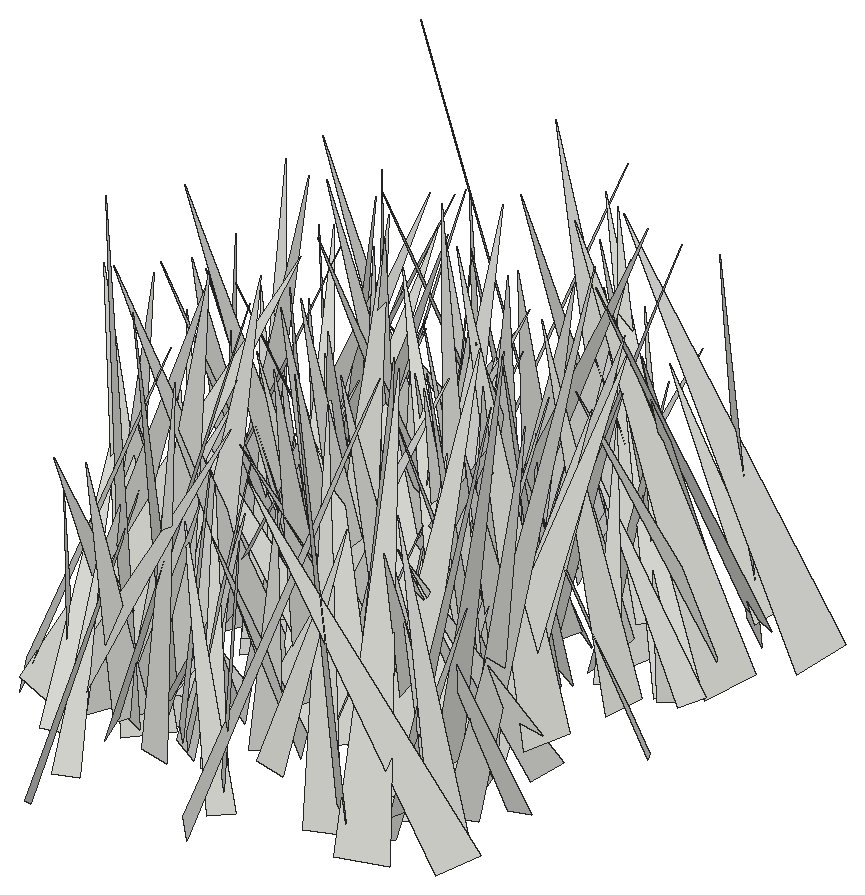
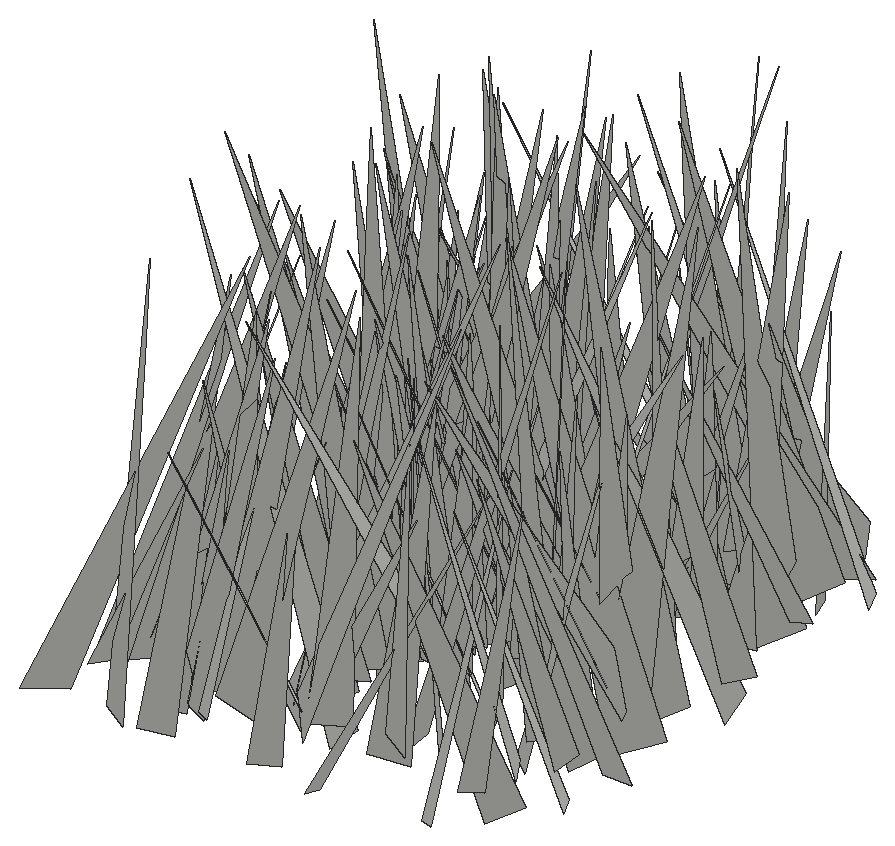
# SketchUp Ruby script. Lengths in inches.
U = 1.inch
M = Sketchup.active_model
def pt(a) = Geom::Point3d.new(a.map { |v| v * U })
def face(e, loops, mat)
  f = e.add_face(loops[0].map { |a| pt(a) })
  loops[1..].each { |l| e.add_face(l.map { |a| pt(a) }).erase! }
  f.material = f.back_material = mat if mat
  f
end
# faces: each face lists its corners as indices into pts; further lists are holes
def faces(e, pts, list, mat = nil) = list.each { |f| face(e, (f[0].is_a?(Array) ? f : [f]).map { |l| l.map { |i| pts[i] } }, mat) }
# xy, xz, yz: faces in a plane at the given z, y or x. An outline is a flat list of corners, or four numbers for a rectangle; further outlines are holes
def ring(l) = l.size == 4 ? [[l[0], l[1]], [l[2], l[1]], [l[2], l[3]], [l[0], l[3]]] : l.each_slice(2).to_a
def flat(e, list, mat, &to3) = list.each { |f| face(e, (f[0].is_a?(Array) ? f : [f]).map { |l| ring(l).map { |u, v| to3.(u, v) } }, mat) }
def xy(e, z, list, mat = nil) = flat(e, list, mat) { |x, y| [x, y, z] }
def xz(e, y, list, mat = nil) = flat(e, list, mat) { |x, z| [x, y, z] }
def yz(e, x, list, mat = nil) = flat(e, list, mat) { |y, z| [x, y, z] }
def lines(e, pts, list) = list.each { |a, b| e.add_line(pt(pts[a]), pt(pts[b])) }
# prism: a flat outline (further loops are holes) pulled along v
def prism(e, loops, v, mat = nil)
  f = face(e, loops, mat); d = Geom::Vector3d.new(v.map { |x| x * U })
  f.pushpull(f.normal.samedirection?(d) ? d.length : -d.length)
end
def box(e, o, s, mat = nil) = prism(e, [[o, [o[0] + s[0], o[1], o[2]], [o[0] + s[0], o[1] + s[1], o[2]], [o[0], o[1] + s[1], o[2]]]], [0, 0, s[2]], mat)
def at(x, y, z, deg = 0) = Geom::Transformation.translation(pt([x, y, z])) * Geom::Transformation.rotation(ORIGIN, Z_AXIS, deg.degrees)
def axes(o, x, y, z) = Geom::Transformation.new([*x, 0, *y, 0, *z, 0, *pt(o).to_a, 1])
def part(name) = M.definitions.add(name)
# library, detail: a bought-in or finely detailed component or shape, given as its bounding box
def library(name, o, s) = part(name).tap { |d| box(d.entities, o, s) }
def detail(e, o, s) = box(e.add_group.entities, o, s)
def put(e, d, t, mat = nil) = e.add_instance(d, t).tap { |i| i.material = mat if mat }
def group(e, t, mat = nil) = e.add_group.tap { |g| g.transformation = t; g.material = mat if mat }.entities
root = M.entities
c1 = part("fur_instance\#9")
p = [[0.8125,0,1.79],[0.67,-0.02,1.48],[0,-0.11,0],[0,0.11,0]]
faces(c1.entities,p,[[0,1,2,3]])
put(root,c1,axes([142.4,106.45,-27.1],[-2.65775,-2.55388,1.91088],[-2.80676,3.05414,0.17806],[1.51521,1.17784,3.68161]))
put(root,c1,axes([137.93,107.84,-27.1],[3.7662,-3.06911,1.25827],[-2.92554,-3.97067,-0.92842],[-1.56328,0.03677,4.76883]))
put(root,c1,axes([137.35,105.55,-28.22],[-2.23531,2.8422,0.49749],[2.78374,2.28983,-0.57415],[0.75919,-0.0278,3.57002]))
put(root,c1,axes([137.45,103.67,-28.22],[4.27823,3.00126,0.70858],[2.21616,-3.83495,2.86263],[-2.14435,2.02448,4.3722]))
put(root,c1,axes([136.09,107.46,-28.22],[-3.74193,-1.93414,1.83822],[-1.95383,4.14237,0.38123],[1.81727,0.47108,4.19495]))
put(root,c1,axes([136.15,106.62,-27.1],[3.52755,5.08967,0.59914],[4.90233,-3.13928,-2.19532],[1.49362,-1.71683,5.79042]))
put(root,c1,axes([139.86,106.47,-27.1],[1.56528,5.39191,1.82425],[5.61252,-1.77733,0.43748],[-0.9488,-1.61836,5.59744]))
put(root,c1,axes([146.14,107.22,-27.1],[3.85266,4.81198,3.39076],[5.17881,-4.69725,0.78179],[-2.79863,-2.06788,6.11449]))
put(root,c1,axes([149.42,108.47,-28.22],[-4.43221,4.72995,1.58971],[4.78005,3.41433,3.16821],[-1.43205,-3.24253,5.65503]))
put(root,c1,axes([142.23,106.57,-28.22],[-1.14245,4.14217,0.46464],[4.01441,0.96381,1.27839],[-1.12161,-0.76952,4.10226]))
put(root,c1,axes([141.9375,105.26,-28.22],[5.64336,5.1887,0.30355],[5.15395,-5.64438,0.66329],[-0.67191,0.28398,7.63742]))
put(root,c1,axes([138.24,109.37,-27.1],[-6.05203,-3.65216,2.90127],[-3.20675,6.70926,1.75646],[3.38709,-0.1736,6.84691]))
put(root,c1,axes([142.83,109.61,-27.1],[-3.8372,-2.33717,0.79383],[-2.01321,3.81242,1.493],[1.42812,-0.90538,4.23762]))
put(root,c1,axes([136.82,105.87,-27.1],[-2.17484,4.53028,0.06229],[4.50087,2.16823,-0.54601],[0.51907,0.1805,4.99552]))
put(root,c1,axes([133.94,107.85,-27.1],[5.98281,3.47845,0.55141],[3.51313,-5.81778,-1.41742],[0.2481,-1.50052,6.77381]))
put(root,c1,axes([137.92,106.97,-27.1],[6.78168,2.91502,1.19431],[2.8839,-6.88568,0.43057],[-1.26762,-0.07012,7.36906]))
put(root,c1,axes([136.63,110.59,-28.22],[3.41213,-4.67618,0.33772],[-4.46229,-3.36731,-1.54031],[-1.43828,-0.64649,5.58003]))
put(root,c1,axes([139.65,107.97,-27.1],[3.10895,3.01642,1.49943],[3.22004,-3.26039,-0.11754],[-0.98914,-1.13301,4.33019]))
put(root,c1,axes([140.05,107.74,-27.1],[3.54809,3.00738,1.07129],[3.07779,-3.64774,0.04651],[-0.84804,-0.65624,4.65093]))
put(root,c1,axes([147.12,106.93,-28.22],[-2.63415,6.93544,1.64719],[7.09873,2.71215,-0.06728],[0.64926,-1.51533,7.41852]))
put(root,c1,axes([142.13,108.77,-27.1],[2.86459,-3.18276,1.27512],[-3.34476,-2.95943,0.1272],[-0.754,1.03614,4.28015]))
put(root,c1,axes([141.63,107.02,-27.1],[-0.67642,4.08917,0.12939],[3.98053,0.62749,0.97839],[-0.94522,-0.2838,4.0276]))
put(root,c1,axes([137.56,108.53,-27.1],[3.65064,-1.60023,0.53489],[-1.66152,-3.63138,0.47591],[-0.29361,0.65299,3.95745]))
put(root,c1,axes([142.9,107.98,-27.1],[0.16923,4.07191,1.2027],[4.12697,0.12503,-1.00402],[0.99752,-1.2081,3.94982]))
put(root,c1,axes([138.05,107.68,-27.1],[3.6249,6.4726,3.15784],[6.5149,-4.45394,1.65071],[-3.06961,-1.8095,7.23254]))
put(root,c1,axes([148.86,108.91,-28.22],[-4.76846,2.17787,1.48985],[2.383,4.8757,0.4998],[1.13316,-1.08876,5.21838]))
put(root,c1,axes([139.09,108.85,-28.22],[1.77196,3.84512,1.4323],[4.08534,-1.50774,-1.0065],[0.38272,-1.70823,4.11239]))
put(root,c1,axes([148.17,109.42,-28.22],[0.92533,-3.44435,1.34936],[-3.58141,-1.18238,-0.56215],[-0.92618,1.13092,3.52189]))
put(root,c1,axes([135.375,108.42,-27.1],[6.77248,-2.83159,1.61361],[-3.13932,-6.6674,1.47599],[-0.87537,2.00399,7.19067]))
put(root,c1,axes([137.61,109.46,-27.1],[5.01911,-5.50348,2.14134],[-5.83765,-5.04831,0.7082],[-0.89193,2.07156,7.41473]))
put(root,c1,axes([145.16,107.55,-28.22],[-0.40472,6.25604,0.83945],[6.18781,0.22712,1.29072],[-1.24649,-0.90382,6.13481]))
put(root,c1,axes([146.9375,108.31,-28.22],[3.77133,0.16267,0.95437],[-0.10228,-3.74984,1.04331],[-0.96272,1.03561,3.6278]))
put(root,c1,axes([137.69,108.92,-28.22],[-4.89648,5.17695,2.06152],[5.4889,4.95404,0.59637],[0.96057,-1.91907,7.10075]))
put(root,c1,axes([145.79,111.78,-28.22],[4.85347,-3.26157,0.26621],[-3.0891,-4.72355,-1.55255],[-1.07988,-1.1468,5.6377]))
put(root,c1,axes([140.43,111.93,-27.1],[-7.65526,-2.65251,1.50577],[-2.23878,7.64939,2.09305],[2.07148,-1.53532,7.82675]))
put(root,c1,axes([135.15,107.2,-27.1],[0.81957,8.13408,0.73803],[7.68253,-0.51597,-2.84467],[2.77248,-0.97476,7.66439]))
put(root,c1,axes([135.86,109.47,-28.22],[6.73151,-1.98165,2.55494],[-2.23492,-7.11595,0.36912],[-2.33662,1.09735,7.00742]))
put(root,c1,axes([141.39,112.16,-27.1],[5.68928,-3.36377,1.44998],[-3.11585,-5.85243,-1.35122],[-1.92583,-0.46842,6.46971]))
put(root,c1,axes([147.45,108.16,-27.1],[5.41894,2.39891,1.8987],[1.67708,-5.5593,2.23748],[-2.55876,1.4367,5.48756]))
put(root,c1,axes([138.29,109.87,-28.22],[-2.68799,6.56885,2.98447],[6.8694,3.30396,-1.08507],[2.20641,-2.2839,7.01411]))
put(root,c1,axes([138.41,108.57,-27.1],[3.83996,1.68055,0.1423],[1.49178,-3.54944,1.66307],[-0.78682,1.47206,3.84756]))
put(root,c1,axes([146.5625,108.91,-27.1],[-1.26821,6.79621,1.34265],[6.86908,1.41065,-0.65215],[0.89826,-1.19212,6.8827]))
put(root,c1,axes([138.6,111.6875,-28.22],[-1.73362,-4.79917,0.85478],[-4.86621,1.65027,-0.60395],[-0.28757,1.00633,5.06683]))
put(root,c1,axes([143.53,111.61,-28.22],[7.52805,-0.18805,1.99939],[0.07054,-7.72753,-0.99239],[-2.00698,-0.97696,7.46472]))
put(root,c1,axes([138.45,109.83,-27.1],[-1.05429,4.67357,0.99792],[4.75005,0.91265,0.74413],[-0.52453,-1.12891,4.73287]))
put(root,c1,axes([137.33,109.22,-27.1],[3.31155,2.43431,1.59522],[1.82743,-3.61986,1.73033],[-2.2652,0.63849,3.72802]))
put(root,c1,axes([138.46,112.3,-28.22],[-3.56897,-0.50146,0.42511],[-0.28446,3.29362,1.49696],[0.59267,-1.43888,3.27843]))
put(root,c1,axes([134.72,110.01,-27.1],[1.36791,4.73736,0.76135],[4.55305,-1.0318,-1.76027],[1.51392,-1.17738,4.60599]))
put(root,c1,axes([144.93,112.41,-28.22],[-6.0404,2.2493,3.21945],[3.13358,6.3206,1.46334],[2.36747,-2.62704,6.2773]))
put(root,c1,axes([148.87,112,-28.22],[-0.83843,-4.56243,0.7415],[-4.45874,0.59959,-1.35228],[-1.2187,0.94513,4.43735]))
put(root,c1,axes([146.85,111.13,-27.1],[7.17764,0.6661,2.04171],[0.73913,-7.45363,-0.1667],[-2.01642,-0.36113,7.20655]))
put(root,c1,axes([143.2,110.18,-27.1],[3.15167,2.15202,0.19961],[2.1362,-3.1554,0.29004],[-0.32814,0.12762,3.80527]))
put(root,c1,axes([146.42,109.5,-28.22],[-3.134,4.47853,0.59876],[4.43295,3.18866,-0.64743],[0.8745,-0.1137,5.42771]))
put(root,c1,axes([142.38,114.28,-27.1],[-4.33714,-4.09832,0.0827],[-3.81397,4.0787,2.10515],[1.50223,-1.4771,5.58349]))
put(root,c1,axes([143.84,110.625,-27.1],[-4.18107,4.06515,1.12452],[4.17237,4.21812,0.26475],[0.61747,-0.97641,5.82552]))
put(root,c1,axes([142.07,113.15,-28.22],[1.08245,-7.41016,1.80762],[-7.58562,-1.23679,-0.52762],[-0.7977,1.70574,7.47019]))
put(root,c1,axes([143.05,113.14,-28.22],[1.42395,-7.42701,2.10024],[-7.62151,-1.69014,-0.80943],[-1.21824,1.89264,7.51884]))
put(root,c1,axes([142.48,112.03,-27.1],[2.08402,3.38406,1.47593],[3.68931,-1.84524,-0.97848],[0.13865,-1.76538,3.85196]))
put(root,c1,axes([141.0625,110.02,-27.1],[2.76171,5.55128,0.00194],[5.48471,-2.72826,-0.95829],[0.85713,-0.42855,6.1258]))
put(root,c1,axes([147.99,114.36,-28.22],[3.38656,-3.48151,1.0277],[-2.77448,-3.38882,-2.33752],[-2.3408,-1.02022,4.25743]))
put(root,c1,axes([138.22,110.84,-27.1],[-1.29816,5.29172,0.79515],[5.27739,1.13069,1.0911],[-0.88529,-1.01932,5.33826]))
put(root,c1,axes([141.62,112.05,-28.22],[-4.37552,-5.12362,2.64469],[-5.63456,4.50416,-0.59611],[1.22377,2.41912,6.71129]))
put(root,c1,axes([147.04,112.95,-28.22],[-6.26815,-2.22604,2.13273],[-2.17784,6.6177,0.5065],[2.18193,0.21043,6.63238]))
put(root,c1,axes([142.6,112.83,-28.22],[-3.83855,4.56526,0.77541],[4.17711,2.97899,3.13921],[-1.99865,-2.54191,5.07163]))
put(root,c1,axes([139.14,111.34,-28.22],[2.58432,3.47984,0.90101],[3.42396,-2.72089,0.68775],[-1.09434,-0.29537,4.2796]))
put(root,c1,axes([146.92,112.56,-28.22],[5.91491,-0.67607,1.90084],[-0.77835,-6.19702,0.21795],[-1.8613,0.44302,5.94943]))
put(root,c1,axes([142.53,111.66,-27.1],[-5.26533,5.42334,2.66225],[5.51698,5.75546,-0.81326],[2.46233,-1.29842,7.51498]))
put(root,c1,axes([138.85,115.84,-28.22],[-6.21102,-4.85766,0.88936],[-4.64444,6.23147,1.60082],[1.67841,-0.73247,7.72082]))
put(root,c1,axes([134.03,113.62,-27.1],[2.085,-4.49657,0.98747],[-4.39792,-1.62495,1.88661],[1.36107,1.63764,4.58334]))
put(root,c1,axes([141.14,113.375,-27.1],[-1.13244,4.66111,1.93868],[4.91983,0.57378,1.4943],[-1.13125,-2.17064,4.55801]))
put(root,c1,axes([139.22,116.12,-27.1],[6.38115,-3.67921,0.2036],[-3.55943,-6.25987,-1.56256],[-0.95316,-1.25481,7.1982]))
put(root,c1,axes([136.625,113.68,-27.1],[-5.78196,-1.74059,3.08913],[-1.82129,6.52793,0.26926],[3.04225,0.59997,6.03227]))
put(root,c1,axes([146.49,112.57,-27.1],[0.66704,7.88186,2.68055],[8.14998,-1.16705,1.40349],[-1.69907,-2.50365,7.78452]))
put(root,c1,axes([142.83,112.1,-28.22],[-6.11447,-3.98639,0.59028],[-3.68819,5.10346,-3.73879],[-1.62389,3.41906,6.26894]))
put(root,c1,axes([142.9375,112.52,-27.1],[1.28068,6.67783,2.12971],[6.86225,-1.63556,1.00185],[-1.42781,-1.87102,6.72532]))
put(root,c1,axes([145.47,112.33,-28.22],[-4.22823,5.63878,0.60494],[5.64653,4.11564,1.10357],[-0.52773,-1.14251,6.96102]))
put(root,c1,axes([146.75,112.27,-27.1],[-4.59485,5.55244,0.46156],[5.5505,4.50971,1.00485],[-0.48434,-0.99407,7.1367]))
put(root,c1,axes([140.03,114.74,-27.1],[-0.48012,-7.554,2.16495],[-7.6037,-0.10085,-2.03814],[-1.98335,2.21526,7.28968]))
put(root,c1,axes([145.87,115.49,-28.22],[-4.57132,-4.01454,0.83204],[-3.89365,4.6413,1.00178],[1.28384,-0.21818,6.00082]))
put(root,c1,axes([146.01,115.48,-27.1],[4.30794,-3.29071,0.86204],[-3.07513,-4.36194,-1.28347],[-1.45447,-0.52435,5.26686]))
put(root,c1,axes([144,111.79,-27.1],[3.8094,4.08661,1.06154],[3.80016,-3.94157,1.53675],[-1.84012,0.32005,5.37125]))
put(root,c1,axes([139.89,115.82,-28.22],[1.13503,-7.67663,0.6742],[-6.50823,-0.58999,4.2389],[4.12651,1.18099,6.50005]))
put(root,c1,axes([137.83,113.67,-27.1],[1.56835,-2.82264,1.69633],[-3.20586,-1.73838,0.07137],[-0.75322,1.52161,3.2283]))
put(root,c1,axes([141.06,111.82,-28.22],[-4.20767,6.2047,0.57896],[6.20765,4.23458,-0.26697],[0.54635,-0.32858,7.49209]))
put(root,c1,axes([144.21,115.25,-27.1],[4.56733,-2.95407,1.62637],[-2.80415,-4.84794,-0.93072],[-1.87305,0.05455,5.35918]))
put(root,c1,axes([146.04,111.3,-28.22],[3.4696,4.95294,0.18512],[4.68916,-3.35343,1.83583],[-1.60551,0.90933,5.7619]))
put(root,c1,axes([142.82,114.63,-28.22],[5.21956,1.10973,1.69595],[1.36173,-5.39042,-0.66376],[-1.50115,-1.03121,5.29478]))
put(root,c1,axes([141.88,116.56,-28.22],[-4.57477,-6.03245,0.25242],[-6.03633,4.57654,-0.02819],[0.13005,0.21817,7.57088]))
put(root,c1,axes([140.39,115.91,-27.1],[7.09602,-3.54407,1.49132],[-3.45875,-7.25092,-0.77408],[-1.67974,-0.04148,7.89397]))
put(root,c1,axes([135.8,116.79,-28.22],[5.76412,-4.56343,1.38579],[-4.26746,-5.90574,-1.69745],[-2.12934,-0.51736,7.15322]))
put(root,c1,axes([147.77,110.66,-28.22],[7.29611,1.84526,3.54482],[-0.04664,-7.33917,3.91643],[-3.99607,3.45479,6.4265]))
put(root,c1,axes([148.15,114.13,-27.1],[-7.39383,1.79038,1.19471],[1.82356,7.48136,0.07416],[1.14343,-0.35412,7.60715]))
put(root,c1,axes([142.66,115.25,-27.1],[4.32257,0.5968,0.21737],[0.63053,-4.21214,-0.97382],[-0.07654,-0.99484,4.25352]))
put(root,c1,axes([144.61,116.51,-27.1],[-1.86183,-7.54983,1.10161],[-7.50699,1.61006,-1.65309],[-1.3633,1.44488,7.59827]))
put(root,c1,axes([134.35,113.41,-28.22],[7.12948,2.21776,0.41944],[2.17259,-7.11974,0.71624],[-0.61174,0.56098,7.43203]))
put(root,c1,axes([146.26,113.17,-28.22],[-2.83058,6.09964,1.95872],[5.76034,3.3604,-2.14023],[2.80369,-0.74599,6.37473]))
put(root,c1,axes([143.7,115.59,-27.1],[-0.98581,-7.65367,2.64082],[-7.9173,0.35473,-1.92744],[-1.69382,2.79641,7.47232]))
put(root,c1,axes([142,115.32,-27.1],[-3.00946,-2.45302,0.73779],[-2.54129,3.00205,-0.38468],[0.32167,0.76736,3.86344]))
put(root,c1,axes([135.63,115.03,-28.22],[7.67247,-2.21843,2.0813],[-2.41925,-7.8734,0.52613],[-1.84403,1.09916,7.96941]))
put(root,c1,axes([143.82,117,-28.22],[2.97455,-6.14482,0.55918],[-6.16848,-2.94679,0.43089],[0.14598,0.69067,6.8133]))
put(root,c1,axes([142.46,115.19,-28.22],[1.70203,4.17643,2.24286],[4.55719,-2.09788,0.44817],[-1.30578,-1.87783,4.48761]))
put(root,c1,axes([145.69,114.27,-28.22],[0.03547,5.69131,1.501],[5.73382,0.30561,-1.29426],[1.32938,-1.46999,5.5423]))
put(root,c1,axes([146.19,114.5,-28.22],[-6.24639,-1.28271,0.8155],[-1.43317,6.11916,-1.35263],[0.50635,1.49608,6.23162]))
put(root,c1,axes([138.42,115.25,-27.1],[7.76844,-0.71206,0.72464],[-0.74639,-7.79129,0.34557],[-0.68922,0.41169,7.79335]))
put(root,c1,axes([142.93,116.97,-28.22],[5.81845,-0.62274,2.18855],[-0.03101,-6.03017,-1.6334],[-2.27522,-1.51035,5.61909]))
put(root,c1,axes([141.45,116.22,-27.1],[1.4619,-3.63585,0.57448],[-3.60479,-1.28901,1.01518],[0.74496,0.89757,3.78497]))
put(root,c1,axes([143.47,115.35,-28.22],[-3.37291,-1.64413,0.77782],[-1.79286,3.28135,-0.83849],[0.30629,1.10194,3.65741]))
put(root,c1,axes([143.64,113.87,-28.22],[-0.24232,8.0833,1.63068],[8.24361,0.27788,-0.15248],[0.20433,-1.625,8.08549]))
put(root,c1,axes([139.07,115.83,-28.22],[-5.46878,-3.64969,2.6695],[-4.02035,5.84198,-0.2491],[2.0696,1.70441,6.57007]))
put(root,c1,axes([137.57,114.96,-27.1],[-1.32199,4.73147,0.88748],[4.77716,1.17578,0.84759],[-0.59431,-1.0737,4.83901]))
put(root,c1,axes([135.05,116.86,-28.22],[5.01421,-5.55154,0.43768],[-5.45899,-4.78379,1.86233],[1.10028,1.565,7.24525]))
put(root,c1,axes([138.72,115.47,-28.22],[-2.00481,-4.221,2.16779],[-4.72189,1.54205,-1.3643],[-0.46899,2.51807,4.46932]))
put(root,c1,axes([136.06,115.38,-27.1],[2.47782,3.1575,0.0552],[3.13992,-2.45577,-0.47176],[0.33732,-0.3344,3.98583]))
put(root,c1,axes([145.11,115.31,-28.22],[3.40494,2.47984,0.75094],[2.39973,-3.48584,0.63038],[-0.97714,0.08048,4.16483]))
put(root,c1,axes([145.12,116.42,-27.1],[-0.35143,6.05342,2.99786],[6.31844,1.35633,-1.99808],[2.38924,-2.69649,5.72495]))
put(root,c1,axes([141.15,116.77,-27.1],[1.68942,-4.24341,1.91691],[-4.60334,-1.82876,0.00876],[-0.70022,1.78447,4.56734]))
put(root,c1,axes([139.01,115.82,-28.22],[4.92095,5.18553,0.33695],[5.09859,-4.72846,-1.69263],[1.00379,-1.4039,6.94554]))
put(root,c1,axes([143.02,115.7,-27.1],[3.50267,-1.34823,2.1537],[-1.97697,-3.75014,0.86764],[-1.59615,1.68627,3.65152]))
put(root,c1,axes([137.29,114.69,-28.22],[-6.65914,2.85732,1.17721],[2.6023,6.69305,-1.52492],[1.66678,0.96593,7.084]))
put(root,c1,axes([143.03,118.36,-27.1],[3.4393,-6.56896,1.063],[-6.65437,-3.3911,0.57422],[0.02233,1.20797,7.39258]))
put(root,c1,axes([149.71,116.87,-28.22],[-3.22375,-2.36609,0.00506],[-2.25529,3.0702,-1.21594],[-0.71558,0.9831,3.80952]))
put(root,c1,axes([143.21,116.65,-27.1],[3.08289,1.97486,1.70839],[2.08981,-3.45082,0.21788],[-1.56569,-0.71742,3.6547]))
put(root,c1,axes([142.81,115.57,-27.1],[-1.16488,5.07104,1.08343],[5.11451,1.30667,-0.61696],[0.85504,-0.90739,5.16641]))
put(root,c1,axes([141.17,117.3,-28.22],[-0.7765,-5.95979,2.50914],[-6.25232,1.3369,1.24057],[1.65027,2.26084,5.88073]))
put(root,c1,axes([137.91,116.87,-28.22],[-5.05567,-0.39861,1.84756],[-0.46846,5.37567,-0.1221],[1.83109,0.27472,5.06989]))
put(root,c1,axes([148.62,117.1,-27.1],[-6.00997,1.04438,1.22572],[1.13938,6.10462,0.38513],[1.13796,-0.59647,6.08787]))
put(root,c1,axes([142.98,116.6,-28.22],[1.148,3.43718,0.90942],[3.54891,-1.0498,-0.51218],[0.21566,-1.0212,3.58745]))
put(root,c1,axes([144.43,119.02,-28.22],[-2.91514,-5.53327,1.42514],[-5.42873,3.18122,1.24695],[1.78243,0.63944,6.12864]))
put(root,c1,axes([136.49,117.46,-28.22],[-0.53957,3.97433,2.02364],[4.38519,0.84425,-0.48882],[0.81275,-1.91664,3.98089]))
put(root,c1,axes([142.8,118.28,-28.22],[3.87563,-0.57439,1.14349],[-0.32332,-3.96837,-0.89752],[-1.23813,-0.76168,3.81378]))
put(root,c1,axes([137.09,115.875,-27.1],[2.95968,3.81178,0.17357],[3.80838,-2.96454,0.16477],[-0.23661,-0.0359,4.82309]))
put(root,c1,axes([138.15,115.27,-27.1],[-2.51338,5.74575,1.01303],[5.46798,2.70448,-1.77311],[2.03497,-0.17044,6.01555]))
put(root,c1,axes([143.37,120.52,-28.22],[5.49992,-4.64771,0.52674],[-4.40214,-5.41809,-1.84207],[-1.58109,-1.08206,6.96111]))
put(root,c1,axes([136.89,118.56,-27.1],[6.91292,1.02767,1.79019],[1.3308,-7.00178,-1.11957],[-1.57792,-1.40299,6.89863]))
put(root,c1,axes([145.31,117.2,-27.1],[1.49909,3.09185,1.25062],[3.12666,-1.78006,0.6529],[-1.16087,-0.8017,3.3735]))
put(root,c1,axes([144.79,119.09,-28.22],[-3.69542,-5.95234,1.80806],[-6.20183,3.68953,-0.52934],[0.48649,1.82006,6.98615]))
put(root,c1,axes([140.57,118.14,-27.1],[1.59272,-3.9303,2.28796],[-4.37909,-1.9795,-0.352],[-1.22702,1.96293,4.22612]))
put(root,c1,axes([137.01,119.6,-28.22],[-3.21192,-3.98216,0.77509],[-3.98629,3.28152,0.34045],[0.75355,0.38579,5.10471]))
put(root,c1,axes([142.07,117.93,-27.1],[7.97011,-1.5942,0.50435],[-1.65185,-7.88792,1.1707],[-0.25934,1.24806,8.04323]))
put(root,c1,axes([147.4375,117.84,-27.1],[-1.47,3.64091,0.87512],[3.73843,1.4809,0.11844],[0.21496,-0.85654,3.92467]))
put(root,c1,axes([139.67,117.77,-28.22],[3.6626,3.70148,0.35684],[3.71844,-3.64024,-0.40601],[0.03906,-0.53912,5.19141]))
put(root,c1,axes([142.48,119.57,-27.1],[1.87666,-6.19619,1.68038],[-6.32701,-1.4881,1.57887],[1.08876,2.03251,6.27868]))
put(root,c1,axes([143.3125,119.77,-28.22],[5.62437,-1.82953,0.08499],[-1.8284,-5.62476,-0.0835],[-0.10665,-0.05312,5.91386]))
put(root,c1,axes([135.65,118.37,-28.22],[4.38543,-2.43855,0.87514],[-2.59033,-4.09309,1.5752],[0.05089,1.80126,4.76417]))
put(root,c1,axes([135.65,116.43,-27.1],[6.20269,2.14266,0.41588],[1.88774,-5.89525,2.21806],[-1.09562,1.97291,6.17613]))
put(root,c1,axes([148.43,121.65,-27.1],[-4.62318,-3.47557,0.41553],[-3.19467,4.47097,1.85217],[1.4305,-1.24775,5.47931]))
put(root,c1,axes([136.17,119.64,-27.1],[2.52401,-3.24586,0.70539],[-3.32076,-2.44552,0.62916],[0.07602,0.94215,4.0633]))
put(root,c1,axes([143.81,121.24,-28.22],[-4.63636,-6.55031,0.51962],[-6.56307,4.58532,-0.75728],[-0.32055,0.86066,7.9893]))
put(root,c1,axes([140.03,120.55,-28.22],[-7.66466,-1.90179,1.421],[-1.79066,7.78455,0.75987],[1.55871,-0.40873,7.86043]))
put(root,c1,axes([138.12,119.16,-27.1],[5.01686,3.02729,2.73746],[3.17963,-5.61852,0.38618],[-2.55892,-1.04628,5.84673]))
put(root,c1,axes([134.4,118.56,-28.22],[2.40606,6.39383,1.08481],[6.38564,-2.13376,-1.58675],[1.13207,-1.55339,6.64473]))
put(root,c1,axes([148.7,120.13,-28.22],[-2.52237,2.99386,0.77548],[2.99232,2.10973,1.58806],[-0.78138,-1.58517,3.57821]))
put(root,c1,axes([139.11,120.5,-28.22],[4.80931,3.10321,2.02961],[3.46778,-4.94111,-0.66234],[-1.31293,-1.68352,5.68513]))
put(root,c1,axes([149,121.5,-28.22],[-7.26006,2.55391,1.83228],[2.95803,7.11093,1.80912],[1.0629,-2.34529,7.48051]))
put(root,c1,axes([146.35,120.17,-27.1],[-3.92472,-1.58946,0.29836],[-1.61245,3.78584,-1.04222],[-0.12416,1.07696,4.10409]))
put(root,c1,axes([142.43,120.3,-27.1],[0.67083,5.9533,2.27987],[6.17356,-0.03505,-1.72498],[1.58958,-2.37626,5.73727]))
put(root,c1,axes([134.85,120.27,-27.1],[4.46137,-0.22154,0.62784],[-0.29219,-4.4737,0.49769],[-0.59824,0.53291,4.43905]))
put(root,c1,axes([145.25,120.1,-28.22],[4.7353,0.6555,1.15241],[0.55235,-4.8611,0.49538],[-1.20525,0.34759,4.75472]))
put(root,c1,axes([148.38,123.55,-27.1],[-2.55623,-6.61752,0.06611],[-6.61278,2.55692,0.25211],[0.25899,-0.02922,7.08959]))
put(root,c1,axes([141.73,121.53,-28.22],[8.09633,1.85359,0.38508],[1.89305,-7.94545,-1.5559],[-0.02113,-1.6027,8.15877]))
put(root,c1,axes([134.57,120.63,-28.22],[4.03846,2.29721,0.25382],[2.30928,-3.98992,-0.63131],[0.09403,-0.6739,4.60302]))
put(root,c1,axes([146.68,122.0625,-28.22],[-5.38028,-3.08502,1.66928],[-3.07413,5.61908,0.47644],[1.68926,0.39986,6.18367]))
put(root,c1,axes([141.33,122.68,-27.1],[3.50702,-4.68842,0.88051],[-4.69288,-3.58696,-0.4079],[-0.85643,0.45629,5.84073]))
put(root,c1,axes([140.04,121.66,-28.22],[1.39978,-5.30319,2.32473],[-5.64349,-1.78474,-0.67328],[-1.29585,2.04412,5.44334]))
put(root,c1,axes([140.27,118.56,-27.1],[5.9455,4.2001,0.21568],[4.05072,-5.81939,1.66213],[-1.13095,1.23699,7.08711]))
put(root,c1,axes([137,123.81,-28.22],[-2.98193,-4.15353,0.46379],[-3.81224,2.9367,1.78925],[1.71281,-0.69483,4.78981]))
put(root,c1,axes([146.07,124.4375,-28.22],[-0.43827,-6.52973,0.002],[-6.42899,0.43186,1.145],[1.14256,-0.07472,6.44348]))
put(root,c1,axes([135.55,122.1,-28.22],[3.57334,-4.4658,0.19156],[-4.12422,-3.19939,2.34597],[1.72363,1.60293,5.21618]))
put(root,c1,axes([148.125,120.35,-28.22],[-6.04879,4.39479,0.23194],[4.40071,6.03643,0.38865],[-0.04117,-0.45072,7.46666]))
put(root,c1,axes([142.3,121.79,-27.1],[-1.49858,-3.44059,1.04989],[-3.40031,0.98374,-1.62968],[-1.17382,1.54281,3.38047]))
put(root,c1,axes([146.47,123.23,-28.22],[1.52104,-3.59534,0.18519],[-3.58042,-1.53172,-0.32978],[-0.37596,0.04131,3.88989]))
put(root,c1,axes([146.16,121.39,-28.22],[-8.05212,1.79962,1.36323],[1.82873,8.16018,0.02927],[1.32393,-0.32629,8.25072]))
put(root,c1,axes([148.1875,119.78,-28.22],[-5.7713,0.32455,0.04644],[0.28097,5.31808,-2.2482],[0.16895,2.24233,5.3253]))
put(root,c1,axes([135.875,123.2,-27.1],[-3.46561,0.71078,2.1355],[1.4755,3.67824,1.17025],[1.69955,-1.74395,3.33859]))
put(root,c1,axes([145.92,121.25,-27.1],[2.97491,-4.25566,3.74848],[-5.0806,-3.88069,-0.37363],[-2.51977,2.80026,5.17891]))
put(root,c1,axes([140.57,124.37,-28.22],[-4.92347,-1.39259,0.14711],[-1.23579,4.5738,1.93769],[0.65861,-1.82825,4.73553]))
put(root,c1,axes([143.96,123.57,-27.1],[-0.89834,-6.55906,1.37521],[-6.65422,0.70817,-0.96916],[-0.7961,1.48213,6.54897]))
put(root,c1,axes([135.64,121.43,-27.1],[4.69542,3.0157,0.91715],[3.05189,-4.76105,0.03053],[-0.78841,-0.46959,5.58037]))
put(root,c1,axes([144.39,124.45,-27.1],[-3.15103,-4.03715,0.66571],[-3.75697,3.18756,1.54769],[1.62077,-0.46003,4.88182]))
put(root,c1,axes([146.27,122.7,-28.22],[0.81184,5.62301,2.88886],[5.96448,-1.64652,1.52868],[-2.09495,-2.50871,5.47179]))
put(root,c1,axes([142.55,124.04,-28.22],[2.96444,-3.24193,0.90441],[-3.19075,-3.09049,-0.61962],[-1.07107,0.23387,4.34903]))
put(root,c1,axes([139.17,122.45,-27.1],[1.89742,4.59885,2.05217],[4.78177,-2.33318,0.8074],[-1.57969,-1.53878,4.90894]))
put(root,c1,axes([150.02,124.41,-28.22],[-7.32197,2.2534,1.35544],[2.57225,6.97064,2.30649],[0.54639,-2.61889,7.30542]))
put(root,c1,axes([142.64,122.35,-27.1],[3.00056,3.161,0.00616],[3.13284,-2.97269,-0.58633],[0.42105,-0.40809,4.31874]))
put(root,c1,axes([147.52,124.44,-28.22],[3.71105,4.69804,3.51461],[5.68502,-3.90755,-0.77947],[-1.45074,-3.29476,5.93598]))
put(root,c1,axes([142.22,122.85,-27.1],[-6.33694,-5.31771,1.42218],[-5.44687,5.74429,-2.79146],[-0.79519,3.03026,7.78734]))
put(root,c1,axes([148.5,123.82,-27.1],[-3.99734,1.08155,0.32432],[1.12476,3.91891,0.79421],[0.09918,-0.85212,4.0642]))
